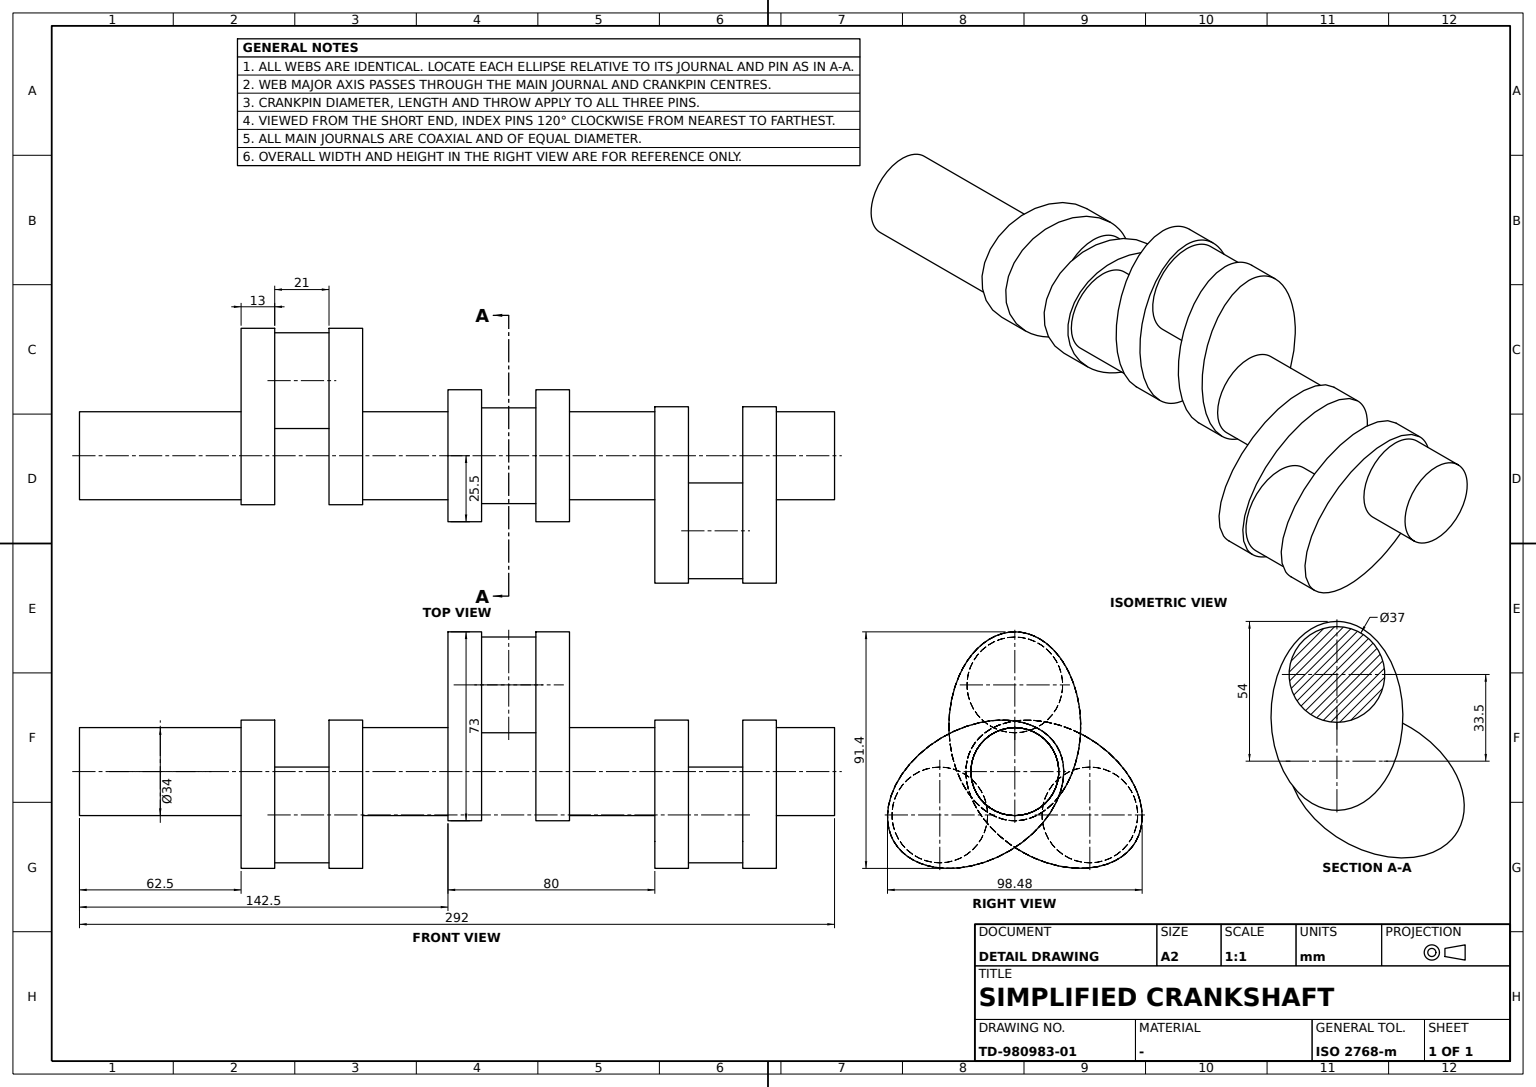
ISO-10303-21;
HEADER;
FILE_DESCRIPTION((''),'2;1');
FILE_NAME('','',(''),(''),'','','');
FILE_SCHEMA(('AUTOMOTIVE_DESIGN'));
ENDSEC;
DATA;
#1=APPLICATION_CONTEXT('');
#2=PRODUCT_CONTEXT('',#1,'mechanical');
#3=PRODUCT('','','',(#2));
#4=PRODUCT_DEFINITION_FORMATION('','',#3);
#5=PRODUCT_DEFINITION_CONTEXT('',#1,'design');
#6=PRODUCT_DEFINITION('','',#4,#5);
#7=PRODUCT_DEFINITION_SHAPE('','',#6);
#8=(LENGTH_UNIT()NAMED_UNIT(*)SI_UNIT(.MILLI.,.METRE.));
#9=(NAMED_UNIT(*)PLANE_ANGLE_UNIT()SI_UNIT($,.RADIAN.));
#10=(NAMED_UNIT(*)SI_UNIT($,.STERADIAN.)SOLID_ANGLE_UNIT());
#11=UNCERTAINTY_MEASURE_WITH_UNIT(LENGTH_MEASURE(0.005),#8,'distance_accuracy_value','');
#12=(GEOMETRIC_REPRESENTATION_CONTEXT(3)GLOBAL_UNCERTAINTY_ASSIGNED_CONTEXT((#11))GLOBAL_UNIT_ASSIGNED_CONTEXT((#8,#9,#10))REPRESENTATION_CONTEXT('',''));
#13=CARTESIAN_POINT('',(0.,33.,-0.5));
#14=VERTEX_POINT('',#13);
#15=CARTESIAN_POINT('',(0.,33.,-17.5));
#16=DIRECTION('',(0.,1.,0.));
#17=DIRECTION('',(0.,0.,1.));
#18=AXIS2_PLACEMENT_3D('',#15,#16,#17);
#19=CIRCLE('',#18,17.);
#20=EDGE_CURVE('',#14,#14,#19,.T.);
#21=ORIENTED_EDGE('',*,*,#20,.F.);
#22=EDGE_LOOP('',(#21));
#23=FACE_BOUND('',#22,.T.);
#24=CARTESIAN_POINT('',(0.,0.,-0.5));
#25=VERTEX_POINT('',#24);
#26=CARTESIAN_POINT('',(0.,0.,-17.5));
#27=AXIS2_PLACEMENT_3D('',#26,#16,#17);
#28=CIRCLE('',#27,17.);
#29=EDGE_CURVE('',#25,#25,#28,.T.);
#30=ORIENTED_EDGE('',*,*,#29,.T.);
#31=EDGE_LOOP('',(#30));
#32=FACE_BOUND('',#31,.T.);
#33=CARTESIAN_POINT('',(0.,-38.25,-17.5));
#34=DIRECTION('',(0.,-1.,0.));
#35=DIRECTION('',(1.,0.,0.));
#36=AXIS2_PLACEMENT_3D('',#33,#34,#35);
#37=CYLINDRICAL_SURFACE('',#36,17.);
#38=ADVANCED_FACE('',(#23,#32),#37,.T.);
#39=CARTESIAN_POINT('',(-29.011851,-13.,-15.75));
#40=VERTEX_POINT('',#39);
#41=CARTESIAN_POINT('',(-29.011851,-13.,-34.25));
#42=AXIS2_PLACEMENT_3D('',#41,#16,#17);
#43=CIRCLE('',#42,18.5);
#44=EDGE_CURVE('',#40,#40,#43,.F.);
#45=ORIENTED_EDGE('',*,*,#44,.F.);
#46=EDGE_LOOP('',(#45));
#47=FACE_BOUND('',#46,.T.);
#48=CARTESIAN_POINT('',(-46.765372,-13.,-44.5));
#49=VERTEX_POINT('',#48);
#50=CARTESIAN_POINT('',(-15.155445,-13.,-26.25));
#51=DIRECTION('',(-0.866025404,0.,-0.5));
#52=AXIS2_PLACEMENT_3D('',#50,#16,#51);
#53=ELLIPSE('',#52,36.5,25.5);
#54=EDGE_CURVE('',#49,#49,#53,.T.);
#55=ORIENTED_EDGE('',*,*,#54,.F.);
#56=EDGE_LOOP('',(#55));
#57=FACE_BOUND('',#56,.T.);
#58=DIRECTION('',(0.5,0.,-0.866025404));
#59=AXIS2_PLACEMENT_3D('',#50,#16,#58);
#60=PLANE('',#59);
#61=ADVANCED_FACE('',(#47,#57),#60,.F.);
#62=CARTESIAN_POINT('',(0.,-109.5,-34.5));
#63=VERTEX_POINT('',#62);
#64=CARTESIAN_POINT('',(0.,-109.5,-17.5));
#65=DIRECTION('',(0.,0.,-1.));
#66=AXIS2_PLACEMENT_3D('',#64,#34,#65);
#67=CIRCLE('',#66,17.);
#68=EDGE_CURVE('',#63,#63,#67,.T.);
#69=ORIENTED_EDGE('',*,*,#68,.T.);
#70=EDGE_LOOP('',(#69));
#71=FACE_BOUND('',#70,.T.);
#72=CARTESIAN_POINT('',(0.,-109.5,0.));
#73=AXIS2_PLACEMENT_3D('',#72,#34,#35);
#74=PLANE('',#73);
#75=ADVANCED_FACE('',(#71),#74,.T.);
#76=CARTESIAN_POINT('',(0.,67.,34.5));
#77=VERTEX_POINT('',#76);
#78=CARTESIAN_POINT('',(0.,67.,16.));
#79=AXIS2_PLACEMENT_3D('',#78,#16,#17);
#80=CIRCLE('',#79,18.5);
#81=EDGE_CURVE('',#77,#77,#80,.F.);
#82=ORIENTED_EDGE('',*,*,#81,.T.);
#83=EDGE_LOOP('',(#82));
#84=FACE_BOUND('',#83,.T.);
#85=CARTESIAN_POINT('',(0.,46.,34.5));
#86=VERTEX_POINT('',#85);
#87=CARTESIAN_POINT('',(0.,46.,16.));
#88=AXIS2_PLACEMENT_3D('',#87,#16,#17);
#89=CIRCLE('',#88,18.5);
#90=EDGE_CURVE('',#86,#86,#89,.F.);
#91=ORIENTED_EDGE('',*,*,#90,.F.);
#92=EDGE_LOOP('',(#91));
#93=FACE_BOUND('',#92,.T.);
#94=CARTESIAN_POINT('',(0.,61.75,16.));
#95=AXIS2_PLACEMENT_3D('',#94,#34,#35);
#96=CYLINDRICAL_SURFACE('',#95,18.5);
#97=ADVANCED_FACE('',(#84,#93),#96,.T.);
#98=CARTESIAN_POINT('',(-46.765372,-34.,-44.5));
#99=VERTEX_POINT('',#98);
#100=CARTESIAN_POINT('',(-15.155445,-34.,-26.25));
#101=AXIS2_PLACEMENT_3D('',#100,#16,#51);
#102=ELLIPSE('',#101,36.5,25.5);
#103=EDGE_CURVE('',#99,#99,#102,.T.);
#104=ORIENTED_EDGE('',*,*,#103,.F.);
#105=EDGE_LOOP('',(#104));
#106=FACE_BOUND('',#105,.T.);
#107=CARTESIAN_POINT('',(-46.765372,-47.,-44.5));
#108=VERTEX_POINT('',#107);
#109=CARTESIAN_POINT('',(-15.155445,-47.,-26.25));
#110=AXIS2_PLACEMENT_3D('',#109,#16,#51);
#111=ELLIPSE('',#110,36.5,25.5);
#112=EDGE_CURVE('',#108,#108,#111,.T.);
#113=ORIENTED_EDGE('',*,*,#112,.T.);
#114=EDGE_LOOP('',(#113));
#115=FACE_BOUND('',#114,.T.);
#116=CARTESIAN_POINT('',(-40.113263,-34.,-52.220818));
#117=CARTESIAN_POINT('',(-40.113263,-47.,-52.220818));
#118=CARTESIAN_POINT('',(-47.588307,-34.,-44.975122));
#119=CARTESIAN_POINT('',(-47.588307,-47.,-44.975122));
#120=CARTESIAN_POINT('',(-50.125742,-34.,-34.878695));
#121=CARTESIAN_POINT('',(-50.125742,-47.,-34.878695));
#122=CARTESIAN_POINT('',(-47.339266,-34.,-23.468629));
#123=CARTESIAN_POINT('',(-47.339266,-47.,-23.468629));
#124=CARTESIAN_POINT('',(-39.653095,-34.,-12.482));
#125=CARTESIAN_POINT('',(-39.653095,-47.,-12.482));
#126=CARTESIAN_POINT('',(-28.237379,-34.,-3.591425));
#127=CARTESIAN_POINT('',(-28.237379,-47.,-3.591425));
#128=CARTESIAN_POINT('',(-14.830057,-34.,1.849587));
#129=CARTESIAN_POINT('',(-14.830057,-47.,1.849587));
#130=CARTESIAN_POINT('',(-1.472272,-34.,3.012692));
#131=CARTESIAN_POINT('',(-1.472272,-47.,3.012692));
#132=CARTESIAN_POINT('',(9.802373,-34.,-0.279182));
#133=CARTESIAN_POINT('',(9.802373,-47.,-0.279182));
#134=CARTESIAN_POINT('',(17.277418,-34.,-7.524878));
#135=CARTESIAN_POINT('',(17.277418,-47.,-7.524878));
#136=CARTESIAN_POINT('',(19.814852,-34.,-17.621305));
#137=CARTESIAN_POINT('',(19.814852,-47.,-17.621305));
#138=CARTESIAN_POINT('',(17.028377,-34.,-29.031371));
#139=CARTESIAN_POINT('',(17.028377,-47.,-29.031371));
#140=CARTESIAN_POINT('',(9.342206,-34.,-40.018));
#141=CARTESIAN_POINT('',(9.342206,-47.,-40.018));
#142=CARTESIAN_POINT('',(-2.07351,-34.,-48.908575));
#143=CARTESIAN_POINT('',(-2.07351,-47.,-48.908575));
#144=CARTESIAN_POINT('',(-15.480832,-34.,-54.349587));
#145=CARTESIAN_POINT('',(-15.480832,-47.,-54.349587));
#146=CARTESIAN_POINT('',(-28.838617,-34.,-55.512692));
#147=CARTESIAN_POINT('',(-28.838617,-47.,-55.512692));
#148=B_SPLINE_SURFACE_WITH_KNOTS('',3,1,((#116,#117),(#118,#119),(#120,#121),(#122,#123),(#124,#125),(#126,#127),(#128,#129),(#130,#131),(#132,#133),(#134,#135),(#136,#137),(#138,#139),(#140,#141),(#142,#143),(#144,#145),(#146,#147),(#116,#117),(#118,#119),(#120,#121)),.SURF_OF_LINEAR_EXTRUSION.,.T.,.F.,.F.,(1,1,1,1,1,1,1,1,1,1,1,1,1,1,1,1,1,1,1,1,1,1,1),(2,2),(-1.178097245,-0.785398163,-0.392699082,0.,0.392699082,0.785398163,1.178097245,1.570796327,1.963495408,2.35619449,2.748893572,3.141592654,3.534291735,3.926990817,4.319689899,4.71238898,5.105088062,5.497787144,5.890486225,6.283185307,6.675884389,7.068583471,7.461282552),(0.,1.),.UNSPECIFIED.);
#149=ADVANCED_FACE('',(#106,#115),#148,.F.);
#150=ORIENTED_EDGE('',*,*,#103,.T.);
#151=EDGE_LOOP('',(#150));
#152=FACE_BOUND('',#151,.T.);
#153=CARTESIAN_POINT('',(-29.011851,-34.,-15.75));
#154=VERTEX_POINT('',#153);
#155=CARTESIAN_POINT('',(-29.011851,-34.,-34.25));
#156=AXIS2_PLACEMENT_3D('',#155,#16,#17);
#157=CIRCLE('',#156,18.5);
#158=EDGE_CURVE('',#154,#154,#157,.F.);
#159=ORIENTED_EDGE('',*,*,#158,.T.);
#160=EDGE_LOOP('',(#159));
#161=FACE_BOUND('',#160,.T.);
#162=AXIS2_PLACEMENT_3D('',#100,#16,#58);
#163=PLANE('',#162);
#164=ADVANCED_FACE('',(#152,#161),#163,.T.);
#165=CARTESIAN_POINT('',(0.,160.,-0.5));
#166=VERTEX_POINT('',#165);
#167=CARTESIAN_POINT('',(0.,160.,-17.5));
#168=AXIS2_PLACEMENT_3D('',#167,#16,#17);
#169=CIRCLE('',#168,17.);
#170=EDGE_CURVE('',#166,#166,#169,.T.);
#171=ORIENTED_EDGE('',*,*,#170,.F.);
#172=EDGE_LOOP('',(#171));
#173=FACE_BOUND('',#172,.T.);
#174=CARTESIAN_POINT('',(46.765372,160.,-44.5));
#175=VERTEX_POINT('',#174);
#176=CARTESIAN_POINT('',(15.155445,160.,-26.25));
#177=DIRECTION('',(0.866025404,0.,-0.5));
#178=AXIS2_PLACEMENT_3D('',#176,#16,#177);
#179=ELLIPSE('',#178,36.5,25.5);
#180=EDGE_CURVE('',#175,#175,#179,.T.);
#181=ORIENTED_EDGE('',*,*,#180,.T.);
#182=EDGE_LOOP('',(#181));
#183=FACE_BOUND('',#182,.T.);
#184=DIRECTION('',(0.5,0.,0.866025404));
#185=AXIS2_PLACEMENT_3D('',#176,#16,#184);
#186=PLANE('',#185);
#187=ADVANCED_FACE('',(#173,#183),#186,.T.);
#188=CARTESIAN_POINT('',(29.011851,126.,-15.75));
#189=VERTEX_POINT('',#188);
#190=CARTESIAN_POINT('',(29.011851,126.,-34.25));
#191=AXIS2_PLACEMENT_3D('',#190,#16,#17);
#192=CIRCLE('',#191,18.5);
#193=EDGE_CURVE('',#189,#189,#192,.F.);
#194=ORIENTED_EDGE('',*,*,#193,.T.);
#195=EDGE_LOOP('',(#194));
#196=FACE_BOUND('',#195,.T.);
#197=CARTESIAN_POINT('',(46.765372,126.,-44.5));
#198=VERTEX_POINT('',#197);
#199=CARTESIAN_POINT('',(15.155445,126.,-26.25));
#200=AXIS2_PLACEMENT_3D('',#199,#16,#177);
#201=ELLIPSE('',#200,36.5,25.5);
#202=EDGE_CURVE('',#198,#198,#201,.T.);
#203=ORIENTED_EDGE('',*,*,#202,.T.);
#204=EDGE_LOOP('',(#203));
#205=FACE_BOUND('',#204,.T.);
#206=AXIS2_PLACEMENT_3D('',#199,#16,#184);
#207=PLANE('',#206);
#208=ADVANCED_FACE('',(#196,#205),#207,.T.);
#209=CARTESIAN_POINT('',(46.765372,147.,-44.5));
#210=VERTEX_POINT('',#209);
#211=CARTESIAN_POINT('',(15.155445,147.,-26.25));
#212=AXIS2_PLACEMENT_3D('',#211,#16,#177);
#213=ELLIPSE('',#212,36.5,25.5);
#214=EDGE_CURVE('',#210,#210,#213,.T.);
#215=ORIENTED_EDGE('',*,*,#214,.F.);
#216=EDGE_LOOP('',(#215));
#217=FACE_BOUND('',#216,.T.);
#218=CARTESIAN_POINT('',(29.011851,147.,-15.75));
#219=VERTEX_POINT('',#218);
#220=CARTESIAN_POINT('',(29.011851,147.,-34.25));
#221=AXIS2_PLACEMENT_3D('',#220,#16,#17);
#222=CIRCLE('',#221,18.5);
#223=EDGE_CURVE('',#219,#219,#222,.F.);
#224=ORIENTED_EDGE('',*,*,#223,.F.);
#225=EDGE_LOOP('',(#224));
#226=FACE_BOUND('',#225,.T.);
#227=AXIS2_PLACEMENT_3D('',#211,#16,#184);
#228=PLANE('',#227);
#229=ADVANCED_FACE('',(#217,#226),#228,.F.);
#230=CARTESIAN_POINT('',(0.,80.,-0.5));
#231=VERTEX_POINT('',#230);
#232=CARTESIAN_POINT('',(0.,80.,-17.5));
#233=AXIS2_PLACEMENT_3D('',#232,#16,#17);
#234=CIRCLE('',#233,17.);
#235=EDGE_CURVE('',#231,#231,#234,.T.);
#236=ORIENTED_EDGE('',*,*,#235,.T.);
#237=EDGE_LOOP('',(#236));
#238=FACE_BOUND('',#237,.T.);
#239=CARTESIAN_POINT('',(0.,113.,-0.5));
#240=VERTEX_POINT('',#239);
#241=CARTESIAN_POINT('',(0.,113.,-17.5));
#242=AXIS2_PLACEMENT_3D('',#241,#16,#17);
#243=CIRCLE('',#242,17.);
#244=EDGE_CURVE('',#240,#240,#243,.T.);
#245=ORIENTED_EDGE('',*,*,#244,.F.);
#246=EDGE_LOOP('',(#245));
#247=FACE_BOUND('',#246,.T.);
#248=ADVANCED_FACE('',(#238,#247),#37,.T.);
#249=ORIENTED_EDGE('',*,*,#44,.T.);
#250=EDGE_LOOP('',(#249));
#251=FACE_BOUND('',#250,.T.);
#252=ORIENTED_EDGE('',*,*,#158,.F.);
#253=EDGE_LOOP('',(#252));
#254=FACE_BOUND('',#253,.T.);
#255=CARTESIAN_POINT('',(-29.011851,-18.25,-34.25));
#256=DIRECTION('',(-0.5,0.,0.866025404));
#257=AXIS2_PLACEMENT_3D('',#255,#34,#256);
#258=CYLINDRICAL_SURFACE('',#257,18.5);
#259=ADVANCED_FACE('',(#251,#254),#258,.T.);
#260=ORIENTED_EDGE('',*,*,#20,.T.);
#261=EDGE_LOOP('',(#260));
#262=FACE_BOUND('',#261,.T.);
#263=CARTESIAN_POINT('',(0.,33.,36.5));
#264=VERTEX_POINT('',#263);
#265=CARTESIAN_POINT('',(0.,33.,0.));
#266=AXIS2_PLACEMENT_3D('',#265,#16,#17);
#267=ELLIPSE('',#266,36.5,25.5);
#268=EDGE_CURVE('',#264,#264,#267,.T.);
#269=ORIENTED_EDGE('',*,*,#268,.F.);
#270=EDGE_LOOP('',(#269));
#271=FACE_BOUND('',#270,.T.);
#272=DIRECTION('',(-1.,0.,0.));
#273=AXIS2_PLACEMENT_3D('',#265,#16,#272);
#274=PLANE('',#273);
#275=ADVANCED_FACE('',(#262,#271),#274,.F.);
#276=ORIENTED_EDGE('',*,*,#214,.T.);
#277=EDGE_LOOP('',(#276));
#278=FACE_BOUND('',#277,.T.);
#279=ORIENTED_EDGE('',*,*,#180,.F.);
#280=EDGE_LOOP('',(#279));
#281=FACE_BOUND('',#280,.T.);
#282=CARTESIAN_POINT('',(50.125742,160.,-34.878695));
#283=CARTESIAN_POINT('',(50.125742,147.,-34.878695));
#284=CARTESIAN_POINT('',(47.588307,160.,-44.975122));
#285=CARTESIAN_POINT('',(47.588307,147.,-44.975122));
#286=CARTESIAN_POINT('',(40.113263,160.,-52.220818));
#287=CARTESIAN_POINT('',(40.113263,147.,-52.220818));
#288=CARTESIAN_POINT('',(28.838617,160.,-55.512692));
#289=CARTESIAN_POINT('',(28.838617,147.,-55.512692));
#290=CARTESIAN_POINT('',(15.480832,160.,-54.349587));
#291=CARTESIAN_POINT('',(15.480832,147.,-54.349587));
#292=CARTESIAN_POINT('',(2.07351,160.,-48.908575));
#293=CARTESIAN_POINT('',(2.07351,147.,-48.908575));
#294=CARTESIAN_POINT('',(-9.342206,160.,-40.018));
#295=CARTESIAN_POINT('',(-9.342206,147.,-40.018));
#296=CARTESIAN_POINT('',(-17.028377,160.,-29.031371));
#297=CARTESIAN_POINT('',(-17.028377,147.,-29.031371));
#298=CARTESIAN_POINT('',(-19.814852,160.,-17.621305));
#299=CARTESIAN_POINT('',(-19.814852,147.,-17.621305));
#300=CARTESIAN_POINT('',(-17.277418,160.,-7.524878));
#301=CARTESIAN_POINT('',(-17.277418,147.,-7.524878));
#302=CARTESIAN_POINT('',(-9.802373,160.,-0.279182));
#303=CARTESIAN_POINT('',(-9.802373,147.,-0.279182));
#304=CARTESIAN_POINT('',(1.472272,160.,3.012692));
#305=CARTESIAN_POINT('',(1.472272,147.,3.012692));
#306=CARTESIAN_POINT('',(14.830057,160.,1.849587));
#307=CARTESIAN_POINT('',(14.830057,147.,1.849587));
#308=CARTESIAN_POINT('',(28.237379,160.,-3.591425));
#309=CARTESIAN_POINT('',(28.237379,147.,-3.591425));
#310=CARTESIAN_POINT('',(39.653095,160.,-12.482));
#311=CARTESIAN_POINT('',(39.653095,147.,-12.482));
#312=CARTESIAN_POINT('',(47.339266,160.,-23.468629));
#313=CARTESIAN_POINT('',(47.339266,147.,-23.468629));
#314=B_SPLINE_SURFACE_WITH_KNOTS('',3,1,((#282,#283),(#284,#285),(#286,#287),(#288,#289),(#290,#291),(#292,#293),(#294,#295),(#296,#297),(#298,#299),(#300,#301),(#302,#303),(#304,#305),(#306,#307),(#308,#309),(#310,#311),(#312,#313),(#282,#283),(#284,#285),(#286,#287)),.SURF_OF_LINEAR_EXTRUSION.,.T.,.F.,.F.,(1,1,1,1,1,1,1,1,1,1,1,1,1,1,1,1,1,1,1,1,1,1,1),(2,2),(-1.178097245,-0.785398163,-0.392699082,0.,0.392699082,0.785398163,1.178097245,1.570796327,1.963495408,2.35619449,2.748893572,3.141592654,3.534291735,3.926990817,4.319689899,4.71238898,5.105088062,5.497787144,5.890486225,6.283185307,6.675884389,7.068583471,7.461282552),(0.,1.),.UNSPECIFIED.);
#315=ADVANCED_FACE('',(#278,#281),#314,.F.);
#316=CARTESIAN_POINT('',(0.,-47.,-0.5));
#317=VERTEX_POINT('',#316);
#318=CARTESIAN_POINT('',(0.,-47.,-17.5));
#319=AXIS2_PLACEMENT_3D('',#318,#16,#17);
#320=CIRCLE('',#319,17.);
#321=EDGE_CURVE('',#317,#317,#320,.T.);
#322=ORIENTED_EDGE('',*,*,#321,.F.);
#323=EDGE_LOOP('',(#322));
#324=FACE_BOUND('',#323,.T.);
#325=ORIENTED_EDGE('',*,*,#68,.F.);
#326=EDGE_LOOP('',(#325));
#327=FACE_BOUND('',#326,.T.);
#328=ADVANCED_FACE('',(#324,#327),#37,.T.);
#329=ORIENTED_EDGE('',*,*,#223,.T.);
#330=EDGE_LOOP('',(#329));
#331=FACE_BOUND('',#330,.T.);
#332=ORIENTED_EDGE('',*,*,#193,.F.);
#333=EDGE_LOOP('',(#332));
#334=FACE_BOUND('',#333,.T.);
#335=CARTESIAN_POINT('',(29.011851,141.75,-34.25));
#336=DIRECTION('',(-0.5,0.,-0.866025404));
#337=AXIS2_PLACEMENT_3D('',#335,#34,#336);
#338=CYLINDRICAL_SURFACE('',#337,18.5);
#339=ADVANCED_FACE('',(#331,#334),#338,.T.);
#340=CARTESIAN_POINT('',(-46.765372,0.,-44.5));
#341=VERTEX_POINT('',#340);
#342=CARTESIAN_POINT('',(-15.155445,0.,-26.25));
#343=AXIS2_PLACEMENT_3D('',#342,#16,#51);
#344=ELLIPSE('',#343,36.5,25.5);
#345=EDGE_CURVE('',#341,#341,#344,.T.);
#346=ORIENTED_EDGE('',*,*,#345,.T.);
#347=EDGE_LOOP('',(#346));
#348=FACE_BOUND('',#347,.T.);
#349=ORIENTED_EDGE('',*,*,#29,.F.);
#350=EDGE_LOOP('',(#349));
#351=FACE_BOUND('',#350,.T.);
#352=AXIS2_PLACEMENT_3D('',#342,#16,#58);
#353=PLANE('',#352);
#354=ADVANCED_FACE('',(#348,#351),#353,.T.);
#355=ORIENTED_EDGE('',*,*,#345,.F.);
#356=EDGE_LOOP('',(#355));
#357=FACE_BOUND('',#356,.T.);
#358=ORIENTED_EDGE('',*,*,#54,.T.);
#359=EDGE_LOOP('',(#358));
#360=FACE_BOUND('',#359,.T.);
#361=CARTESIAN_POINT('',(-40.113263,0.,-52.220818));
#362=CARTESIAN_POINT('',(-40.113263,-13.,-52.220818));
#363=CARTESIAN_POINT('',(-47.588307,0.,-44.975122));
#364=CARTESIAN_POINT('',(-47.588307,-13.,-44.975122));
#365=CARTESIAN_POINT('',(-50.125742,0.,-34.878695));
#366=CARTESIAN_POINT('',(-50.125742,-13.,-34.878695));
#367=CARTESIAN_POINT('',(-47.339266,0.,-23.468629));
#368=CARTESIAN_POINT('',(-47.339266,-13.,-23.468629));
#369=CARTESIAN_POINT('',(-39.653095,0.,-12.482));
#370=CARTESIAN_POINT('',(-39.653095,-13.,-12.482));
#371=CARTESIAN_POINT('',(-28.237379,0.,-3.591425));
#372=CARTESIAN_POINT('',(-28.237379,-13.,-3.591425));
#373=CARTESIAN_POINT('',(-14.830057,0.,1.849587));
#374=CARTESIAN_POINT('',(-14.830057,-13.,1.849587));
#375=CARTESIAN_POINT('',(-1.472272,0.,3.012692));
#376=CARTESIAN_POINT('',(-1.472272,-13.,3.012692));
#377=CARTESIAN_POINT('',(9.802373,0.,-0.279182));
#378=CARTESIAN_POINT('',(9.802373,-13.,-0.279182));
#379=CARTESIAN_POINT('',(17.277418,0.,-7.524878));
#380=CARTESIAN_POINT('',(17.277418,-13.,-7.524878));
#381=CARTESIAN_POINT('',(19.814852,0.,-17.621305));
#382=CARTESIAN_POINT('',(19.814852,-13.,-17.621305));
#383=CARTESIAN_POINT('',(17.028377,0.,-29.031371));
#384=CARTESIAN_POINT('',(17.028377,-13.,-29.031371));
#385=CARTESIAN_POINT('',(9.342206,0.,-40.018));
#386=CARTESIAN_POINT('',(9.342206,-13.,-40.018));
#387=CARTESIAN_POINT('',(-2.07351,0.,-48.908575));
#388=CARTESIAN_POINT('',(-2.07351,-13.,-48.908575));
#389=CARTESIAN_POINT('',(-15.480832,0.,-54.349587));
#390=CARTESIAN_POINT('',(-15.480832,-13.,-54.349587));
#391=CARTESIAN_POINT('',(-28.838617,0.,-55.512692));
#392=CARTESIAN_POINT('',(-28.838617,-13.,-55.512692));
#393=B_SPLINE_SURFACE_WITH_KNOTS('',3,1,((#361,#362),(#363,#364),(#365,#366),(#367,#368),(#369,#370),(#371,#372),(#373,#374),(#375,#376),(#377,#378),(#379,#380),(#381,#382),(#383,#384),(#385,#386),(#387,#388),(#389,#390),(#391,#392),(#361,#362),(#363,#364),(#365,#366)),.SURF_OF_LINEAR_EXTRUSION.,.T.,.F.,.F.,(1,1,1,1,1,1,1,1,1,1,1,1,1,1,1,1,1,1,1,1,1,1,1),(2,2),(-1.178097245,-0.785398163,-0.392699082,0.,0.392699082,0.785398163,1.178097245,1.570796327,1.963495408,2.35619449,2.748893572,3.141592654,3.534291735,3.926990817,4.319689899,4.71238898,5.105088062,5.497787144,5.890486225,6.283185307,6.675884389,7.068583471,7.461282552),(0.,1.),.UNSPECIFIED.);
#394=ADVANCED_FACE('',(#357,#360),#393,.F.);
#395=CARTESIAN_POINT('',(0.,182.5,-34.5));
#396=VERTEX_POINT('',#395);
#397=CARTESIAN_POINT('',(0.,182.5,-17.5));
#398=AXIS2_PLACEMENT_3D('',#397,#34,#65);
#399=CIRCLE('',#398,17.);
#400=EDGE_CURVE('',#396,#396,#399,.T.);
#401=ORIENTED_EDGE('',*,*,#400,.T.);
#402=EDGE_LOOP('',(#401));
#403=FACE_BOUND('',#402,.T.);
#404=ORIENTED_EDGE('',*,*,#170,.T.);
#405=EDGE_LOOP('',(#404));
#406=FACE_BOUND('',#405,.T.);
#407=ADVANCED_FACE('',(#403,#406),#37,.T.);
#408=CARTESIAN_POINT('',(0.,46.,36.5));
#409=VERTEX_POINT('',#408);
#410=CARTESIAN_POINT('',(0.,46.,0.));
#411=AXIS2_PLACEMENT_3D('',#410,#16,#17);
#412=ELLIPSE('',#411,36.5,25.5);
#413=EDGE_CURVE('',#409,#409,#412,.T.);
#414=ORIENTED_EDGE('',*,*,#413,.T.);
#415=EDGE_LOOP('',(#414));
#416=FACE_BOUND('',#415,.T.);
#417=ORIENTED_EDGE('',*,*,#90,.T.);
#418=EDGE_LOOP('',(#417));
#419=FACE_BOUND('',#418,.T.);
#420=AXIS2_PLACEMENT_3D('',#410,#16,#272);
#421=PLANE('',#420);
#422=ADVANCED_FACE('',(#416,#419),#421,.T.);
#423=CARTESIAN_POINT('',(46.765372,113.,-44.5));
#424=VERTEX_POINT('',#423);
#425=CARTESIAN_POINT('',(15.155445,113.,-26.25));
#426=AXIS2_PLACEMENT_3D('',#425,#16,#177);
#427=ELLIPSE('',#426,36.5,25.5);
#428=EDGE_CURVE('',#424,#424,#427,.T.);
#429=ORIENTED_EDGE('',*,*,#428,.T.);
#430=EDGE_LOOP('',(#429));
#431=FACE_BOUND('',#430,.T.);
#432=ORIENTED_EDGE('',*,*,#202,.F.);
#433=EDGE_LOOP('',(#432));
#434=FACE_BOUND('',#433,.T.);
#435=CARTESIAN_POINT('',(50.125742,126.,-34.878695));
#436=CARTESIAN_POINT('',(50.125742,113.,-34.878695));
#437=CARTESIAN_POINT('',(47.588307,126.,-44.975122));
#438=CARTESIAN_POINT('',(47.588307,113.,-44.975122));
#439=CARTESIAN_POINT('',(40.113263,126.,-52.220818));
#440=CARTESIAN_POINT('',(40.113263,113.,-52.220818));
#441=CARTESIAN_POINT('',(28.838617,126.,-55.512692));
#442=CARTESIAN_POINT('',(28.838617,113.,-55.512692));
#443=CARTESIAN_POINT('',(15.480832,126.,-54.349587));
#444=CARTESIAN_POINT('',(15.480832,113.,-54.349587));
#445=CARTESIAN_POINT('',(2.07351,126.,-48.908575));
#446=CARTESIAN_POINT('',(2.07351,113.,-48.908575));
#447=CARTESIAN_POINT('',(-9.342206,126.,-40.018));
#448=CARTESIAN_POINT('',(-9.342206,113.,-40.018));
#449=CARTESIAN_POINT('',(-17.028377,126.,-29.031371));
#450=CARTESIAN_POINT('',(-17.028377,113.,-29.031371));
#451=CARTESIAN_POINT('',(-19.814852,126.,-17.621305));
#452=CARTESIAN_POINT('',(-19.814852,113.,-17.621305));
#453=CARTESIAN_POINT('',(-17.277418,126.,-7.524878));
#454=CARTESIAN_POINT('',(-17.277418,113.,-7.524878));
#455=CARTESIAN_POINT('',(-9.802373,126.,-0.279182));
#456=CARTESIAN_POINT('',(-9.802373,113.,-0.279182));
#457=CARTESIAN_POINT('',(1.472272,126.,3.012692));
#458=CARTESIAN_POINT('',(1.472272,113.,3.012692));
#459=CARTESIAN_POINT('',(14.830057,126.,1.849587));
#460=CARTESIAN_POINT('',(14.830057,113.,1.849587));
#461=CARTESIAN_POINT('',(28.237379,126.,-3.591425));
#462=CARTESIAN_POINT('',(28.237379,113.,-3.591425));
#463=CARTESIAN_POINT('',(39.653095,126.,-12.482));
#464=CARTESIAN_POINT('',(39.653095,113.,-12.482));
#465=CARTESIAN_POINT('',(47.339266,126.,-23.468629));
#466=CARTESIAN_POINT('',(47.339266,113.,-23.468629));
#467=B_SPLINE_SURFACE_WITH_KNOTS('',3,1,((#435,#436),(#437,#438),(#439,#440),(#441,#442),(#443,#444),(#445,#446),(#447,#448),(#449,#450),(#451,#452),(#453,#454),(#455,#456),(#457,#458),(#459,#460),(#461,#462),(#463,#464),(#465,#466),(#435,#436),(#437,#438),(#439,#440)),.SURF_OF_LINEAR_EXTRUSION.,.T.,.F.,.F.,(1,1,1,1,1,1,1,1,1,1,1,1,1,1,1,1,1,1,1,1,1,1,1),(2,2),(-1.178097245,-0.785398163,-0.392699082,0.,0.392699082,0.785398163,1.178097245,1.570796327,1.963495408,2.35619449,2.748893572,3.141592654,3.534291735,3.926990817,4.319689899,4.71238898,5.105088062,5.497787144,5.890486225,6.283185307,6.675884389,7.068583471,7.461282552),(0.,1.),.UNSPECIFIED.);
#468=ADVANCED_FACE('',(#431,#434),#467,.F.);
#469=CARTESIAN_POINT('',(0.,80.,36.5));
#470=VERTEX_POINT('',#469);
#471=CARTESIAN_POINT('',(0.,80.,0.));
#472=AXIS2_PLACEMENT_3D('',#471,#16,#17);
#473=ELLIPSE('',#472,36.5,25.5);
#474=EDGE_CURVE('',#470,#470,#473,.T.);
#475=ORIENTED_EDGE('',*,*,#474,.F.);
#476=EDGE_LOOP('',(#475));
#477=FACE_BOUND('',#476,.T.);
#478=CARTESIAN_POINT('',(0.,67.,36.5));
#479=VERTEX_POINT('',#478);
#480=CARTESIAN_POINT('',(0.,67.,0.));
#481=AXIS2_PLACEMENT_3D('',#480,#16,#17);
#482=ELLIPSE('',#481,36.5,25.5);
#483=EDGE_CURVE('',#479,#479,#482,.T.);
#484=ORIENTED_EDGE('',*,*,#483,.T.);
#485=EDGE_LOOP('',(#484));
#486=FACE_BOUND('',#485,.T.);
#487=CARTESIAN_POINT('',(-10.012479,80.,34.599513));
#488=CARTESIAN_POINT('',(-10.012479,67.,34.599513));
#489=CARTESIAN_POINT('',(0.,80.,37.450243));
#490=CARTESIAN_POINT('',(0.,67.,37.450243));
#491=CARTESIAN_POINT('',(10.012479,80.,34.599513));
#492=CARTESIAN_POINT('',(10.012479,67.,34.599513));
#493=CARTESIAN_POINT('',(18.500649,80.,26.481321));
#494=CARTESIAN_POINT('',(18.500649,67.,26.481321));
#495=CARTESIAN_POINT('',(24.172263,80.,14.331588));
#496=CARTESIAN_POINT('',(24.172263,67.,14.331588));
#497=CARTESIAN_POINT('',(26.163869,80.,0.));
#498=CARTESIAN_POINT('',(26.163869,67.,0.));
#499=CARTESIAN_POINT('',(24.172263,80.,-14.331588));
#500=CARTESIAN_POINT('',(24.172263,67.,-14.331588));
#501=CARTESIAN_POINT('',(18.500649,80.,-26.481321));
#502=CARTESIAN_POINT('',(18.500649,67.,-26.481321));
#503=CARTESIAN_POINT('',(10.012479,80.,-34.599513));
#504=CARTESIAN_POINT('',(10.012479,67.,-34.599513));
#505=CARTESIAN_POINT('',(0.,80.,-37.450243));
#506=CARTESIAN_POINT('',(0.,67.,-37.450243));
#507=CARTESIAN_POINT('',(-10.012479,80.,-34.599513));
#508=CARTESIAN_POINT('',(-10.012479,67.,-34.599513));
#509=CARTESIAN_POINT('',(-18.500649,80.,-26.481321));
#510=CARTESIAN_POINT('',(-18.500649,67.,-26.481321));
#511=CARTESIAN_POINT('',(-24.172263,80.,-14.331588));
#512=CARTESIAN_POINT('',(-24.172263,67.,-14.331588));
#513=CARTESIAN_POINT('',(-26.163869,80.,0.));
#514=CARTESIAN_POINT('',(-26.163869,67.,0.));
#515=CARTESIAN_POINT('',(-24.172263,80.,14.331588));
#516=CARTESIAN_POINT('',(-24.172263,67.,14.331588));
#517=CARTESIAN_POINT('',(-18.500649,80.,26.481321));
#518=CARTESIAN_POINT('',(-18.500649,67.,26.481321));
#519=B_SPLINE_SURFACE_WITH_KNOTS('',3,1,((#487,#488),(#489,#490),(#491,#492),(#493,#494),(#495,#496),(#497,#498),(#499,#500),(#501,#502),(#503,#504),(#505,#506),(#507,#508),(#509,#510),(#511,#512),(#513,#514),(#515,#516),(#517,#518),(#487,#488),(#489,#490),(#491,#492)),.SURF_OF_LINEAR_EXTRUSION.,.T.,.F.,.F.,(1,1,1,1,1,1,1,1,1,1,1,1,1,1,1,1,1,1,1,1,1,1,1),(2,2),(-1.178097245,-0.785398163,-0.392699082,0.,0.392699082,0.785398163,1.178097245,1.570796327,1.963495408,2.35619449,2.748893572,3.141592654,3.534291735,3.926990817,4.319689899,4.71238898,5.105088062,5.497787144,5.890486225,6.283185307,6.675884389,7.068583471,7.461282552),(0.,1.),.UNSPECIFIED.);
#520=ADVANCED_FACE('',(#477,#486),#519,.F.);
#521=ORIENTED_EDGE('',*,*,#268,.T.);
#522=EDGE_LOOP('',(#521));
#523=FACE_BOUND('',#522,.T.);
#524=ORIENTED_EDGE('',*,*,#413,.F.);
#525=EDGE_LOOP('',(#524));
#526=FACE_BOUND('',#525,.T.);
#527=CARTESIAN_POINT('',(-10.012479,46.,34.599513));
#528=CARTESIAN_POINT('',(-10.012479,33.,34.599513));
#529=CARTESIAN_POINT('',(0.,46.,37.450243));
#530=CARTESIAN_POINT('',(0.,33.,37.450243));
#531=CARTESIAN_POINT('',(10.012479,46.,34.599513));
#532=CARTESIAN_POINT('',(10.012479,33.,34.599513));
#533=CARTESIAN_POINT('',(18.500649,46.,26.481321));
#534=CARTESIAN_POINT('',(18.500649,33.,26.481321));
#535=CARTESIAN_POINT('',(24.172263,46.,14.331588));
#536=CARTESIAN_POINT('',(24.172263,33.,14.331588));
#537=CARTESIAN_POINT('',(26.163869,46.,0.));
#538=CARTESIAN_POINT('',(26.163869,33.,0.));
#539=CARTESIAN_POINT('',(24.172263,46.,-14.331588));
#540=CARTESIAN_POINT('',(24.172263,33.,-14.331588));
#541=CARTESIAN_POINT('',(18.500649,46.,-26.481321));
#542=CARTESIAN_POINT('',(18.500649,33.,-26.481321));
#543=CARTESIAN_POINT('',(10.012479,46.,-34.599513));
#544=CARTESIAN_POINT('',(10.012479,33.,-34.599513));
#545=CARTESIAN_POINT('',(0.,46.,-37.450243));
#546=CARTESIAN_POINT('',(0.,33.,-37.450243));
#547=CARTESIAN_POINT('',(-10.012479,46.,-34.599513));
#548=CARTESIAN_POINT('',(-10.012479,33.,-34.599513));
#549=CARTESIAN_POINT('',(-18.500649,46.,-26.481321));
#550=CARTESIAN_POINT('',(-18.500649,33.,-26.481321));
#551=CARTESIAN_POINT('',(-24.172263,46.,-14.331588));
#552=CARTESIAN_POINT('',(-24.172263,33.,-14.331588));
#553=CARTESIAN_POINT('',(-26.163869,46.,0.));
#554=CARTESIAN_POINT('',(-26.163869,33.,0.));
#555=CARTESIAN_POINT('',(-24.172263,46.,14.331588));
#556=CARTESIAN_POINT('',(-24.172263,33.,14.331588));
#557=CARTESIAN_POINT('',(-18.500649,46.,26.481321));
#558=CARTESIAN_POINT('',(-18.500649,33.,26.481321));
#559=B_SPLINE_SURFACE_WITH_KNOTS('',3,1,((#527,#528),(#529,#530),(#531,#532),(#533,#534),(#535,#536),(#537,#538),(#539,#540),(#541,#542),(#543,#544),(#545,#546),(#547,#548),(#549,#550),(#551,#552),(#553,#554),(#555,#556),(#557,#558),(#527,#528),(#529,#530),(#531,#532)),.SURF_OF_LINEAR_EXTRUSION.,.T.,.F.,.F.,(1,1,1,1,1,1,1,1,1,1,1,1,1,1,1,1,1,1,1,1,1,1,1),(2,2),(-1.178097245,-0.785398163,-0.392699082,0.,0.392699082,0.785398163,1.178097245,1.570796327,1.963495408,2.35619449,2.748893572,3.141592654,3.534291735,3.926990817,4.319689899,4.71238898,5.105088062,5.497787144,5.890486225,6.283185307,6.675884389,7.068583471,7.461282552),(0.,1.),.UNSPECIFIED.);
#560=ADVANCED_FACE('',(#523,#526),#559,.F.);
#561=ORIENTED_EDGE('',*,*,#428,.F.);
#562=EDGE_LOOP('',(#561));
#563=FACE_BOUND('',#562,.T.);
#564=ORIENTED_EDGE('',*,*,#244,.T.);
#565=EDGE_LOOP('',(#564));
#566=FACE_BOUND('',#565,.T.);
#567=AXIS2_PLACEMENT_3D('',#425,#16,#184);
#568=PLANE('',#567);
#569=ADVANCED_FACE('',(#563,#566),#568,.F.);
#570=ORIENTED_EDGE('',*,*,#321,.T.);
#571=EDGE_LOOP('',(#570));
#572=FACE_BOUND('',#571,.T.);
#573=ORIENTED_EDGE('',*,*,#112,.F.);
#574=EDGE_LOOP('',(#573));
#575=FACE_BOUND('',#574,.T.);
#576=AXIS2_PLACEMENT_3D('',#109,#16,#58);
#577=PLANE('',#576);
#578=ADVANCED_FACE('',(#572,#575),#577,.F.);
#579=ORIENTED_EDGE('',*,*,#235,.F.);
#580=EDGE_LOOP('',(#579));
#581=FACE_BOUND('',#580,.T.);
#582=ORIENTED_EDGE('',*,*,#474,.T.);
#583=EDGE_LOOP('',(#582));
#584=FACE_BOUND('',#583,.T.);
#585=AXIS2_PLACEMENT_3D('',#471,#16,#272);
#586=PLANE('',#585);
#587=ADVANCED_FACE('',(#581,#584),#586,.T.);
#588=ORIENTED_EDGE('',*,*,#81,.F.);
#589=EDGE_LOOP('',(#588));
#590=FACE_BOUND('',#589,.T.);
#591=ORIENTED_EDGE('',*,*,#483,.F.);
#592=EDGE_LOOP('',(#591));
#593=FACE_BOUND('',#592,.T.);
#594=AXIS2_PLACEMENT_3D('',#480,#16,#272);
#595=PLANE('',#594);
#596=ADVANCED_FACE('',(#590,#593),#595,.F.);
#597=ORIENTED_EDGE('',*,*,#400,.F.);
#598=EDGE_LOOP('',(#597));
#599=FACE_BOUND('',#598,.T.);
#600=CARTESIAN_POINT('',(0.,182.5,0.));
#601=AXIS2_PLACEMENT_3D('',#600,#34,#35);
#602=PLANE('',#601);
#603=ADVANCED_FACE('',(#599),#602,.F.);
#604=CLOSED_SHELL('',(#38,#61,#75,#97,#149,#164,#187,#208,#229,#248,#259,#275,#315,#328,#339,#354,#394,#407,#422,#468,#520,#560,#569,#578,#587,#596,#603));
#605=MANIFOLD_SOLID_BREP('',#604);
#606=ADVANCED_BREP_SHAPE_REPRESENTATION('',(#605),#12);
#607=SHAPE_DEFINITION_REPRESENTATION(#7,#606);
ENDSEC;
END-ISO-10303-21;
